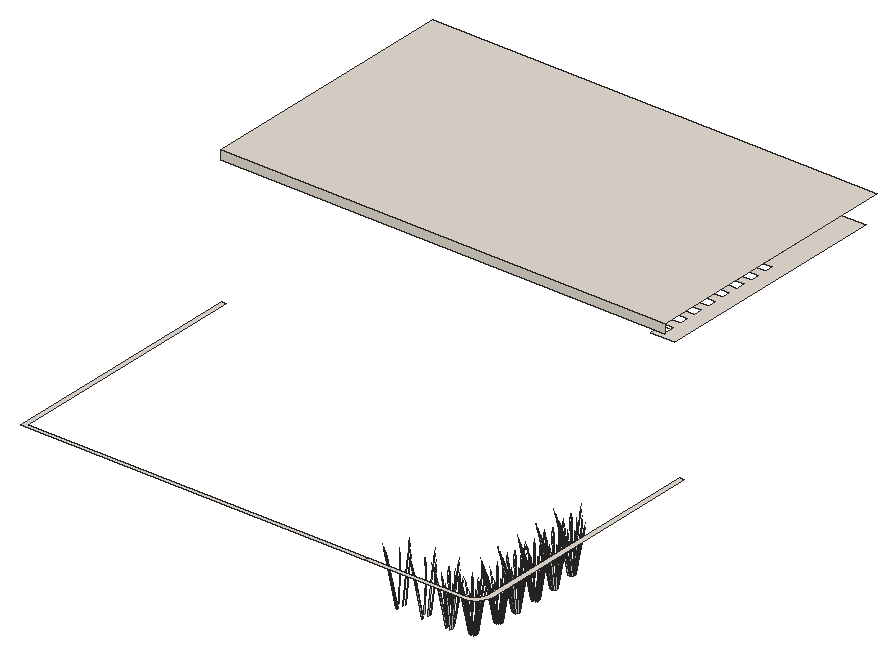
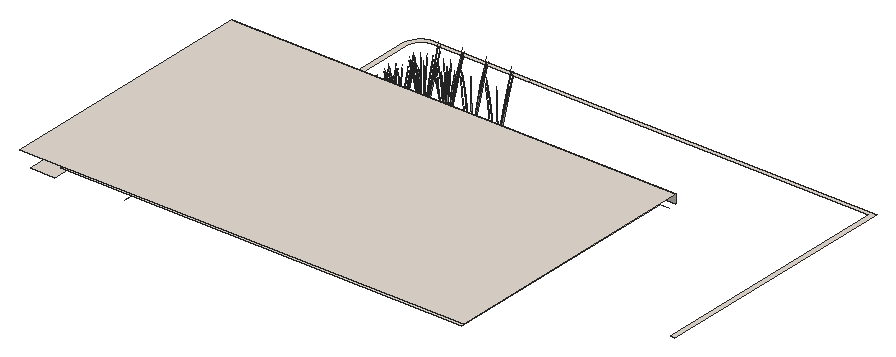
# SketchUp Ruby script. Lengths in inches.
U = 1.inch
M = Sketchup.active_model
def pt(a) = Geom::Point3d.new(a.map { |v| v * U })
def face(e, loops, mat)
  f = e.add_face(loops[0].map { |a| pt(a) })
  loops[1..].each { |l| e.add_face(l.map { |a| pt(a) }).erase! }
  f.material = f.back_material = mat if mat
  f
end
# faces: each face lists its corners as indices into pts; further lists are holes
def faces(e, pts, list, mat = nil) = list.each { |f| face(e, (f[0].is_a?(Array) ? f : [f]).map { |l| l.map { |i| pts[i] } }, mat) }
# xy, xz, yz: faces in a plane at the given z, y or x. An outline is a flat list of corners, or four numbers for a rectangle; further outlines are holes
def ring(l) = l.size == 4 ? [[l[0], l[1]], [l[2], l[1]], [l[2], l[3]], [l[0], l[3]]] : l.each_slice(2).to_a
def flat(e, list, mat, &to3) = list.each { |f| face(e, (f[0].is_a?(Array) ? f : [f]).map { |l| ring(l).map { |u, v| to3.(u, v) } }, mat) }
def xy(e, z, list, mat = nil) = flat(e, list, mat) { |x, y| [x, y, z] }
def xz(e, y, list, mat = nil) = flat(e, list, mat) { |x, z| [x, y, z] }
def yz(e, x, list, mat = nil) = flat(e, list, mat) { |y, z| [x, y, z] }
def lines(e, pts, list) = list.each { |a, b| e.add_line(pt(pts[a]), pt(pts[b])) }
# prism: a flat outline (further loops are holes) pulled along v
def prism(e, loops, v, mat = nil)
  f = face(e, loops, mat); d = Geom::Vector3d.new(v.map { |x| x * U })
  f.pushpull(f.normal.samedirection?(d) ? d.length : -d.length)
end
def box(e, o, s, mat = nil) = prism(e, [[o, [o[0] + s[0], o[1], o[2]], [o[0] + s[0], o[1] + s[1], o[2]], [o[0], o[1] + s[1], o[2]]]], [0, 0, s[2]], mat)
def at(x, y, z, deg = 0) = Geom::Transformation.translation(pt([x, y, z])) * Geom::Transformation.rotation(ORIGIN, Z_AXIS, deg.degrees)
def axes(o, x, y, z) = Geom::Transformation.new([*x, 0, *y, 0, *z, 0, *pt(o).to_a, 1])
def part(name) = M.definitions.add(name)
# library, detail: a bought-in or finely detailed component or shape, given as its bounding box
def library(name, o, s) = part(name).tap { |d| box(d.entities, o, s) }
def detail(e, o, s) = box(e.add_group.entities, o, s)
def put(e, d, t, mat = nil) = e.add_instance(d, t).tap { |i| i.material = mat if mat }
def group(e, t, mat = nil) = e.add_group.tap { |g| g.transformation = t; g.material = mat if mat }.entities
root = M.entities
M.materials.add("LightPink_Translucent").color = [144, 107, 117]
M.materials["LightPink_Translucent"].alpha = 0.75
M.materials.add("Marble_01_1K").color = [230, 221, 211]
c1 = part("blade")
p = [[2.15,0.21,22],[0,0.17,0],[0.09,0.45,0],[2.18,0.31,22],[2.29,0.31,22],[0.38,0.45,0],
  [2.48,0.24,33],[2.49,0.24,33],[2.48,0.22,33]]
faces(c1.entities,p,[[0,1,2,3],[4,5,2,3],[6,3,4,7],[8,0,3,6]])
c2 = part("seeds")
p = [[0.3,-0.1,1.38],[-0.01,-0.03,1.59],[-0.01,-0.03,0.03],[0.14,-0.07,-0.07],[0.29,-0.03,3],[0.15,0.01,3.11]]
faces(c2.entities,p,[[0,1,2,3],[1,0,4,5]],"LightPink_Translucent")
c3 = part("blade with seeds")
put(c3.entities,c1,at(0,0,0))
put(c3.entities,c2,axes([2.4,0.25,30.99],[1.5799,-0.05474,1.17369],[-0.12525,1.92788,0.29478],[-0.07173,-0.02425,1.56792]))
xy(root,300,[[39,42,273,42,273,45,42,45,42,213,39,213],[273,42,339,42,340.56,42.125,342.09,42.45,343.56,42.97,344.96,43.67,346.25,44.54,347.42,45.58,348.46,46.75,349.33,48.04,350.03,49.44,350.55,50.91,350.875,52.44,351,54,351,216,348,216,348,54.05,347.9,52.875,347.66,51.72,347.27,50.61,346.74,49.56,346.08,48.58,345.3,47.7,344.42,46.92,343.44,46.26,342.39,45.73,341.28,45.34,340.125,45.1,338.95,45,273,45]],"Marble_01_1K")
xy(root,375,[[321,225,321,231,327,231,327,237,321,237,321,243,327,243,327,249,321,249,321,255,327,255,327,261,321,261,321,267,327,267,327,273,321,273,321,279,327,279,327,285,321,285,321,291,327,291,327,297,321,297,321,303,327,303,327,309,321,309,321,315,327,315,327,321,321,321,321,387,337.5,387,337.5,225]],"Marble_01_1K")
xy(root,384,[[267,216,273,222],[42,222,315,390]],"Marble_01_1K")
xy(root,390,[[36,216,337.5,396]],"Marble_01_1K")
xz(root,216,[[36,384,337.5,390]],"Marble_01_1K")
p = [[267,390,384],[267,396,384],[42,222,384],[36,222,384],[315,222,384],[337.5,222,384]]
lines(root,p,[[0,1],[2,3],[4,5]])
put(root,c3,axes([317.74,58.68,268.7],[0.34603,-0.28618,0.32977],[0.32756,0.32677,-0.42575],[-0.04984,0.16603,0.81462]))
put(root,c3,axes([317.14,57.8,268.7],[0.44516,-0.07768,0.32977],[0.11755,0.44407,-0.42575],[-0.12757,0.11927,0.81462]))
put(root,c3,axes([319.79,59.08,268.7],[-0.07899,-0.43781,0.32977],[0.45153,-0.11561,-0.42575],[0.12128,0.12546,0.81462]))
put(root,c3,axes([321.1,56.48,268.7],[-0.44516,0.07768,0.32977],[-0.11755,-0.44407,-0.42575],[0.12757,-0.11927,0.81462]))
put(root,c3,axes([317.07,56.74,268.7],[0.42502,0.15163,0.32977],[-0.12396,0.44238,-0.42575],[-0.17112,0.04056,0.81462]))
put(root,c3,axes([320.5,55.59,268.7],[-0.34603,0.28618,0.32977],[-0.32756,-0.32677,-0.42575],[0.04984,-0.16603,0.81462]))
put(root,c3,axes([318.45,55.19,268.7],[0.07899,0.43781,0.32977],[-0.45153,0.11561,-0.42575],[-0.12128,-0.12546,0.81462]))
put(root,c3,axes([332.55,61.85,268.7],[0.15418,-0.41799,0.32977],[0.44981,0.12192,-0.42575],[0.04124,0.16829,0.81462]))
put(root,c3,axes([333.36,57.82,268.7],[-0.15418,0.41799,0.32977],[-0.44981,-0.12192,-0.42575],[-0.04124,-0.16829,0.81462]))
put(root,c3,axes([334.52,61.19,268.7],[-0.29098,-0.34031,0.32977],[0.33226,-0.32215,-0.42575],[0.16881,0.04902,0.81462]))
put(root,c3,axes([335,60.24,268.7],[-0.42502,-0.15163,0.32977],[0.12396,-0.44238,-0.42575],[0.17112,-0.04056,0.81462]))
put(root,c3,axes([331.38,58.48,268.7],[0.29098,0.34031,0.32977],[-0.33226,0.32215,-0.42575],[-0.16881,-0.04902,0.81462]))
put(root,c3,axes([331.57,61.38,268.7],[0.34603,-0.28618,0.32977],[0.32756,0.32677,-0.42575],[-0.04984,0.16603,0.81462]))
put(root,c3,axes([330.97,60.5,268.7],[0.44516,-0.07768,0.32977],[0.11755,0.44407,-0.42575],[-0.12757,0.11927,0.81462]))
put(root,c3,axes([333.625,61.78,268.7],[-0.07899,-0.43781,0.32977],[0.45153,-0.11561,-0.42575],[0.12128,0.12546,0.81462]))
put(root,c3,axes([334.93,59.17,268.7],[-0.44516,0.07768,0.32977],[-0.11755,-0.44407,-0.42575],[0.12757,-0.11927,0.81462]))
put(root,c3,axes([330.9,59.43,268.7],[0.42502,0.15163,0.32977],[-0.12396,0.44238,-0.42575],[-0.17112,0.04056,0.81462]))
put(root,c3,axes([334.33,58.29,268.7],[-0.34603,0.28618,0.32977],[-0.32756,-0.32677,-0.42575],[0.04984,-0.16603,0.81462]))
put(root,c3,axes([332.28,57.89,268.7],[0.07899,0.43781,0.32977],[-0.45153,0.11561,-0.42575],[-0.12128,-0.12546,0.81462]))
put(root,c3,axes([335.24,79.7,268.7],[0.15418,-0.41799,0.32977],[0.44981,0.12192,-0.42575],[0.04124,0.16829,0.81462]))
put(root,c3,axes([336.06,75.67,268.7],[-0.15418,0.41799,0.32977],[-0.44981,-0.12192,-0.42575],[-0.04124,-0.16829,0.81462]))
put(root,c3,axes([337.22,79.04,268.7],[-0.29098,-0.34031,0.32977],[0.33226,-0.32215,-0.42575],[0.16881,0.04902,0.81462]))
put(root,c3,axes([337.7,78.09,268.7],[-0.42502,-0.15163,0.32977],[0.12396,-0.44238,-0.42575],[0.17112,-0.04056,0.81462]))
put(root,c3,axes([334.08,76.33,268.7],[0.29098,0.34031,0.32977],[-0.33226,0.32215,-0.42575],[-0.16881,-0.04902,0.81462]))
put(root,c3,axes([334.27,79.23,268.7],[0.34603,-0.28618,0.32977],[0.32756,0.32677,-0.42575],[-0.04984,0.16603,0.81462]))
put(root,c3,axes([333.67,78.35,268.7],[0.44516,-0.07768,0.32977],[0.11755,0.44407,-0.42575],[-0.12757,0.11927,0.81462]))
put(root,c3,axes([336.32,79.63,268.7],[-0.07899,-0.43781,0.32977],[0.45153,-0.11561,-0.42575],[0.12128,0.12546,0.81462]))
put(root,c3,axes([337.63,77.02,268.7],[-0.44516,0.07768,0.32977],[-0.11755,-0.44407,-0.42575],[0.12757,-0.11927,0.81462]))
put(root,c3,axes([333.6,77.28,268.7],[0.42502,0.15163,0.32977],[-0.12396,0.44238,-0.42575],[-0.17112,0.04056,0.81462]))
put(root,c3,axes([337.03,76.14,268.7],[-0.34603,0.28618,0.32977],[-0.32756,-0.32677,-0.42575],[0.04984,-0.16603,0.81462]))
put(root,c3,axes([334.98,75.74,268.7],[0.07899,0.43781,0.32977],[-0.45153,0.11561,-0.42575],[-0.12128,-0.12546,0.81462]))
put(root,c3,axes([335.24,94.59,268.7],[0.15418,-0.41799,0.32977],[0.44981,0.12192,-0.42575],[0.04124,0.16829,0.81462]))
put(root,c3,axes([336.06,90.56,268.7],[-0.15418,0.41799,0.32977],[-0.44981,-0.12192,-0.42575],[-0.04124,-0.16829,0.81462]))
put(root,c3,axes([337.22,93.93,268.7],[-0.29098,-0.34031,0.32977],[0.33226,-0.32215,-0.42575],[0.16881,0.04902,0.81462]))
put(root,c3,axes([337.7,92.97,268.7],[-0.42502,-0.15163,0.32977],[0.12396,-0.44238,-0.42575],[0.17112,-0.04056,0.81462]))
put(root,c3,axes([334.08,91.22,268.7],[0.29098,0.34031,0.32977],[-0.33226,0.32215,-0.42575],[-0.16881,-0.04902,0.81462]))
put(root,c3,axes([334.27,94.12,268.7],[0.34603,-0.28618,0.32977],[0.32756,0.32677,-0.42575],[-0.04984,0.16603,0.81462]))
put(root,c3,axes([333.67,93.23,268.7],[0.44516,-0.07768,0.32977],[0.11755,0.44407,-0.42575],[-0.12757,0.11927,0.81462]))
put(root,c3,axes([336.32,94.52,268.7],[-0.07899,-0.43781,0.32977],[0.45153,-0.11561,-0.42575],[0.12128,0.12546,0.81462]))
put(root,c3,axes([337.63,91.91,268.7],[-0.44516,0.07768,0.32977],[-0.11755,-0.44407,-0.42575],[0.12757,-0.11927,0.81462]))
put(root,c3,axes([333.6,92.17,268.7],[0.42502,0.15163,0.32977],[-0.12396,0.44238,-0.42575],[-0.17112,0.04056,0.81462]))
put(root,c3,axes([337.03,91.03,268.7],[-0.34603,0.28618,0.32977],[-0.32756,-0.32677,-0.42575],[0.04984,-0.16603,0.81462]))
put(root,c3,axes([334.98,90.625,268.7],[0.07899,0.43781,0.32977],[-0.45153,0.11561,-0.42575],[-0.12128,-0.12546,0.81462]))
put(root,c3,axes([335.24,111.01,268.7],[0.15418,-0.41799,0.32977],[0.44981,0.12192,-0.42575],[0.04124,0.16829,0.81462]))
put(root,c3,axes([336.06,106.97,268.7],[-0.15418,0.41799,0.32977],[-0.44981,-0.12192,-0.42575],[-0.04124,-0.16829,0.81462]))
put(root,c3,axes([337.22,110.34,268.7],[-0.29098,-0.34031,0.32977],[0.33226,-0.32215,-0.42575],[0.16881,0.04902,0.81462]))
put(root,c3,axes([337.7,109.39,268.7],[-0.42502,-0.15163,0.32977],[0.12396,-0.44238,-0.42575],[0.17112,-0.04056,0.81462]))
put(root,c3,axes([334.08,107.63,268.7],[0.29098,0.34031,0.32977],[-0.33226,0.32215,-0.42575],[-0.16881,-0.04902,0.81462]))
put(root,c3,axes([334.27,110.53,268.7],[0.34603,-0.28618,0.32977],[0.32756,0.32677,-0.42575],[-0.04984,0.16603,0.81462]))
put(root,c3,axes([333.67,109.65,268.7],[0.44516,-0.07768,0.32977],[0.11755,0.44407,-0.42575],[-0.12757,0.11927,0.81462]))
put(root,c3,axes([336.32,110.9375,268.7],[-0.07899,-0.43781,0.32977],[0.45153,-0.11561,-0.42575],[0.12128,0.12546,0.81462]))
put(root,c3,axes([337.63,108.33,268.7],[-0.44516,0.07768,0.32977],[-0.11755,-0.44407,-0.42575],[0.12757,-0.11927,0.81462]))
put(root,c3,axes([333.6,108.59,268.7],[0.42502,0.15163,0.32977],[-0.12396,0.44238,-0.42575],[-0.17112,0.04056,0.81462]))
put(root,c3,axes([337.03,107.44,268.7],[-0.34603,0.28618,0.32977],[-0.32756,-0.32677,-0.42575],[0.04984,-0.16603,0.81462]))
put(root,c3,axes([334.98,107.04,268.7],[0.07899,0.43781,0.32977],[-0.45153,0.11561,-0.42575],[-0.12128,-0.12546,0.81462]))
put(root,c3,axes([335.24,126.84,268.7],[0.15418,-0.41799,0.32977],[0.44981,0.12192,-0.42575],[0.04124,0.16829,0.81462]))
put(root,c3,axes([336.06,122.8125,268.7],[-0.15418,0.41799,0.32977],[-0.44981,-0.12192,-0.42575],[-0.04124,-0.16829,0.81462]))
put(root,c3,axes([337.22,126.18,268.7],[-0.29098,-0.34031,0.32977],[0.33226,-0.32215,-0.42575],[0.16881,0.04902,0.81462]))
put(root,c3,axes([337.7,125.23,268.7],[-0.42502,-0.15163,0.32977],[0.12396,-0.44238,-0.42575],[0.17112,-0.04056,0.81462]))
put(root,c3,axes([334.08,123.47,268.7],[0.29098,0.34031,0.32977],[-0.33226,0.32215,-0.42575],[-0.16881,-0.04902,0.81462]))
put(root,c3,axes([334.27,126.375,268.7],[0.34603,-0.28618,0.32977],[0.32756,0.32677,-0.42575],[-0.04984,0.16603,0.81462]))
put(root,c3,axes([333.67,125.49,268.7],[0.44516,-0.07768,0.32977],[0.11755,0.44407,-0.42575],[-0.12757,0.11927,0.81462]))
put(root,c3,axes([336.32,126.78,268.7],[-0.07899,-0.43781,0.32977],[0.45153,-0.11561,-0.42575],[0.12128,0.12546,0.81462]))
put(root,c3,axes([337.63,124.17,268.7],[-0.44516,0.07768,0.32977],[-0.11755,-0.44407,-0.42575],[0.12757,-0.11927,0.81462]))
put(root,c3,axes([333.6,124.43,268.7],[0.42502,0.15163,0.32977],[-0.12396,0.44238,-0.42575],[-0.17112,0.04056,0.81462]))
put(root,c3,axes([337.03,123.28,268.7],[-0.34603,0.28618,0.32977],[-0.32756,-0.32677,-0.42575],[0.04984,-0.16603,0.81462]))
put(root,c3,axes([334.98,122.88,268.7],[0.07899,0.43781,0.32977],[-0.45153,0.11561,-0.42575],[-0.12128,-0.12546,0.81462]))
put(root,c3,axes([333.03,144.85,268.7],[0.15418,-0.41799,0.32977],[0.44981,0.12192,-0.42575],[0.04124,0.16829,0.81462]))
put(root,c3,axes([333.84,140.82,268.7],[-0.15418,0.41799,0.32977],[-0.44981,-0.12192,-0.42575],[-0.04124,-0.16829,0.81462]))
put(root,c3,axes([335.01,144.19,268.7],[-0.29098,-0.34031,0.32977],[0.33226,-0.32215,-0.42575],[0.16881,0.04902,0.81462]))
put(root,c3,axes([335.48,143.24,268.7],[-0.42502,-0.15163,0.32977],[0.12396,-0.44238,-0.42575],[0.17112,-0.04056,0.81462]))
put(root,c3,axes([331.86,141.48,268.7],[0.29098,0.34031,0.32977],[-0.33226,0.32215,-0.42575],[-0.16881,-0.04902,0.81462]))
put(root,c3,axes([332.06,144.38,268.7],[0.34603,-0.28618,0.32977],[0.32756,0.32677,-0.42575],[-0.04984,0.16603,0.81462]))
put(root,c3,axes([331.45,143.5,268.7],[0.44516,-0.07768,0.32977],[0.11755,0.44407,-0.42575],[-0.12757,0.11927,0.81462]))
put(root,c3,axes([334.11,144.79,268.7],[-0.07899,-0.43781,0.32977],[0.45153,-0.11561,-0.42575],[0.12128,0.12546,0.81462]))
put(root,c3,axes([335.41,142.18,268.7],[-0.44516,0.07768,0.32977],[-0.11755,-0.44407,-0.42575],[0.12757,-0.11927,0.81462]))
put(root,c3,axes([331.38,142.4375,268.7],[0.42502,0.15163,0.32977],[-0.12396,0.44238,-0.42575],[-0.17112,0.04056,0.81462]))
put(root,c3,axes([334.8125,141.29,268.7],[-0.34603,0.28618,0.32977],[-0.32756,-0.32677,-0.42575],[0.04984,-0.16603,0.81462]))
put(root,c3,axes([332.76,140.89,268.7],[0.07899,0.43781,0.32977],[-0.45153,0.11561,-0.42575],[-0.12128,-0.12546,0.81462]))
put(root,c3,axes([285.125,59.5,268.72],[-0.50393,-0.1421,0.49617],[0.17232,-0.46717,0.40911],[0.03028,0.18372,1.0267]))
put(root,c3,axes([302.34,59.5,268.72],[-0.50393,-0.1421,0.49617],[0.17232,-0.46717,0.40911],[0.03028,0.18372,1.0267]))
put(root,c3,axes([318.71,59.5,268.72],[-0.50393,-0.1421,0.49617],[0.17232,-0.46717,0.40911],[0.03028,0.18372,1.0267]))
put(root,c3,axes([332.54,62.19,268.72],[-0.50393,-0.1421,0.49617],[0.17232,-0.46717,0.40911],[0.03028,0.18372,1.0267]))
put(root,c3,axes([335.24,80.04,268.72],[-0.50393,-0.1421,0.49617],[0.17232,-0.46717,0.40911],[0.03028,0.18372,1.0267]))
put(root,c3,axes([335.24,94.93,268.72],[-0.50393,-0.1421,0.49617],[0.17232,-0.46717,0.40911],[0.03028,0.18372,1.0267]))
put(root,c3,axes([335.24,111.35,268.72],[-0.50393,-0.1421,0.49617],[0.17232,-0.46717,0.40911],[0.03028,0.18372,1.0267]))
put(root,c3,axes([335.24,127.1875,268.72],[-0.50393,-0.1421,0.49617],[0.17232,-0.46717,0.40911],[0.03028,0.18372,1.0267]))
put(root,c3,axes([333.02,145.2,268.72],[-0.50393,-0.1421,0.49617],[0.17232,-0.46717,0.40911],[0.03028,0.18372,1.0267]))
put(root,c3,axes([283.51,55.48,268.74],[0.42234,-0.40113,0.50064],[0.36424,0.42599,0.4128],[-0.19815,-0.07399,1.03595]))
put(root,c3,axes([284.66,54.68,268.74],[0.56969,-0.13971,0.50064],[0.09887,0.54803,0.4128],[-0.13398,-0.16152,1.03595]))
put(root,c3,axes([300.73,55.48,268.74],[0.42234,-0.40113,0.50064],[0.36424,0.42599,0.4128],[-0.19815,-0.07399,1.03595]))
put(root,c3,axes([301.88,54.68,268.74],[0.56969,-0.13971,0.50064],[0.09887,0.54803,0.4128],[-0.13398,-0.16152,1.03595]))
put(root,c3,axes([317.09,55.48,268.74],[0.42234,-0.40113,0.50064],[0.36424,0.42599,0.4128],[-0.19815,-0.07399,1.03595]))
put(root,c3,axes([318.25,54.68,268.74],[0.56969,-0.13971,0.50064],[0.09887,0.54803,0.4128],[-0.13398,-0.16152,1.03595]))
put(root,c3,axes([330.93,58.17,268.74],[0.42234,-0.40113,0.50064],[0.36424,0.42599,0.4128],[-0.19815,-0.07399,1.03595]))
put(root,c3,axes([332.08,57.375,268.74],[0.56969,-0.13971,0.50064],[0.09887,0.54803,0.4128],[-0.13398,-0.16152,1.03595]))
put(root,c3,axes([333.62,76.02,268.74],[0.42234,-0.40113,0.50064],[0.36424,0.42599,0.4128],[-0.19815,-0.07399,1.03595]))
put(root,c3,axes([334.78,75.22,268.74],[0.56969,-0.13971,0.50064],[0.09887,0.54803,0.4128],[-0.13398,-0.16152,1.03595]))
put(root,c3,axes([333.62,90.91,268.74],[0.42234,-0.40113,0.50064],[0.36424,0.42599,0.4128],[-0.19815,-0.07399,1.03595]))
put(root,c3,axes([334.78,90.11,268.74],[0.56969,-0.13971,0.50064],[0.09887,0.54803,0.4128],[-0.13398,-0.16152,1.03595]))
put(root,c3,axes([333.62,107.33,268.74],[0.42234,-0.40113,0.50064],[0.36424,0.42599,0.4128],[-0.19815,-0.07399,1.03595]))
put(root,c3,axes([334.78,106.53,268.74],[0.56969,-0.13971,0.50064],[0.09887,0.54803,0.4128],[-0.13398,-0.16152,1.03595]))
put(root,c3,axes([333.62,123.17,268.74],[0.42234,-0.40113,0.50064],[0.36424,0.42599,0.4128],[-0.19815,-0.07399,1.03595]))
put(root,c3,axes([334.78,122.37,268.74],[0.56969,-0.13971,0.50064],[0.09887,0.54803,0.4128],[-0.13398,-0.16152,1.03595]))
put(root,c3,axes([331.41,141.18,268.74],[0.42234,-0.40113,0.50064],[0.36424,0.42599,0.4128],[-0.19815,-0.07399,1.03595]))
put(root,c3,axes([332.56,140.375,268.74],[0.56969,-0.13971,0.50064],[0.09887,0.54803,0.4128],[-0.13398,-0.16152,1.03595]))
put(root,c3,axes([285.74,60.65,269.26],[0.35341,-0.31182,-0.06041],[0.32382,0.34152,-0.27392],[0.0228,0.09677,0.90349]))
put(root,c3,axes([282.55,59.06,269.26],[0.45129,0.14509,-0.06041],[-0.13882,0.44656,-0.27392],[-0.07381,0.0678,0.90349]))
put(root,c3,axes([302.95,60.65,269.26],[0.35341,-0.31182,-0.06041],[0.32382,0.34152,-0.27392],[0.0228,0.09677,0.90349]))
put(root,c3,axes([299.77,59.06,269.26],[0.45129,0.14509,-0.06041],[-0.13882,0.44656,-0.27392],[-0.07381,0.0678,0.90349]))
put(root,c3,axes([319.32,60.65,269.26],[0.35341,-0.31182,-0.06041],[0.32382,0.34152,-0.27392],[0.0228,0.09677,0.90349]))
put(root,c3,axes([316.13,59.06,269.26],[0.45129,0.14509,-0.06041],[-0.13882,0.44656,-0.27392],[-0.07381,0.0678,0.90349]))
put(root,c3,axes([333.15,63.34,269.26],[0.35341,-0.31182,-0.06041],[0.32382,0.34152,-0.27392],[0.0228,0.09677,0.90349]))
put(root,c3,axes([329.96,61.76,269.26],[0.45129,0.14509,-0.06041],[-0.13882,0.44656,-0.27392],[-0.07381,0.0678,0.90349]))
put(root,c3,axes([335.85,81.19,269.26],[0.35341,-0.31182,-0.06041],[0.32382,0.34152,-0.27392],[0.0228,0.09677,0.90349]))
put(root,c3,axes([332.66,79.61,269.26],[0.45129,0.14509,-0.06041],[-0.13882,0.44656,-0.27392],[-0.07381,0.0678,0.90349]))
put(root,c3,axes([335.85,96.08,269.26],[0.35341,-0.31182,-0.06041],[0.32382,0.34152,-0.27392],[0.0228,0.09677,0.90349]))
put(root,c3,axes([332.66,94.49,269.26],[0.45129,0.14509,-0.06041],[-0.13882,0.44656,-0.27392],[-0.07381,0.0678,0.90349]))
put(root,c3,axes([335.85,112.5,269.26],[0.35341,-0.31182,-0.06041],[0.32382,0.34152,-0.27392],[0.0228,0.09677,0.90349]))
put(root,c3,axes([332.66,110.91,269.26],[0.45129,0.14509,-0.06041],[-0.13882,0.44656,-0.27392],[-0.07381,0.0678,0.90349]))
put(root,c3,axes([335.85,128.34,269.26],[0.35341,-0.31182,-0.06041],[0.32382,0.34152,-0.27392],[0.0228,0.09677,0.90349]))
put(root,c3,axes([332.66,126.75,269.26],[0.45129,0.14509,-0.06041],[-0.13882,0.44656,-0.27392],[-0.07381,0.0678,0.90349]))
put(root,c3,axes([333.63,146.35,269.26],[0.35341,-0.31182,-0.06041],[0.32382,0.34152,-0.27392],[0.0228,0.09677,0.90349]))
put(root,c3,axes([330.44,144.76,269.26],[0.45129,0.14509,-0.06041],[-0.13882,0.44656,-0.27392],[-0.07381,0.0678,0.90349]))
